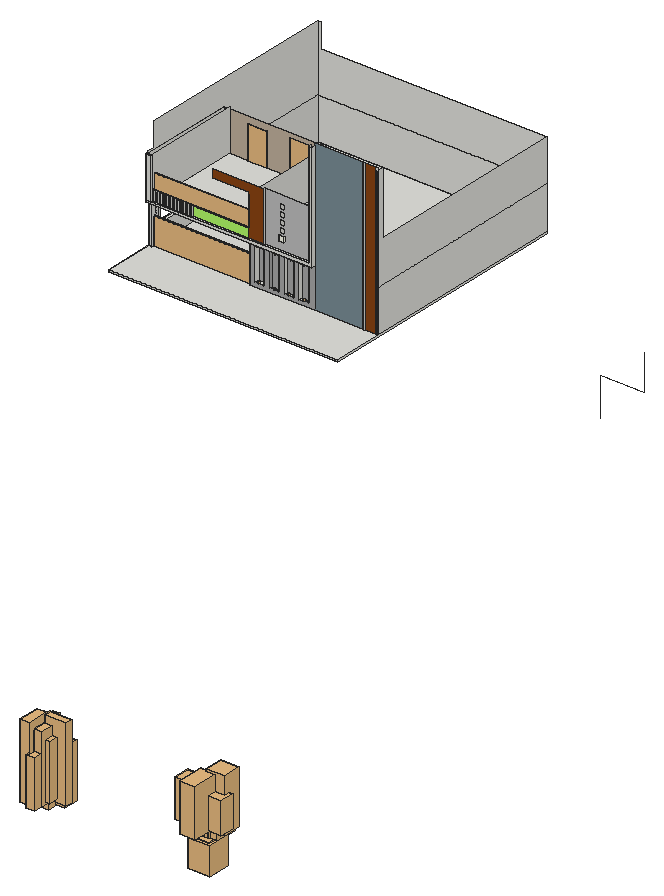
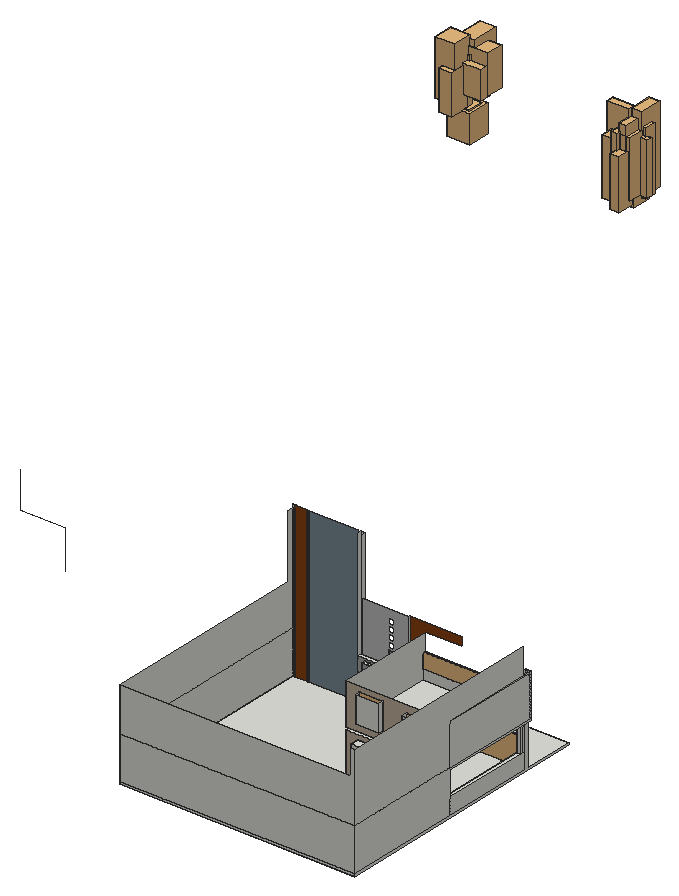
# SketchUp Ruby script. Lengths in inches.
U = 1.inch
M = Sketchup.active_model
def pt(a) = Geom::Point3d.new(a.map { |v| v * U })
def face(e, loops, mat)
  f = e.add_face(loops[0].map { |a| pt(a) })
  loops[1..].each { |l| e.add_face(l.map { |a| pt(a) }).erase! }
  f.material = f.back_material = mat if mat
  f
end
# faces: each face lists its corners as indices into pts; further lists are holes
def faces(e, pts, list, mat = nil) = list.each { |f| face(e, (f[0].is_a?(Array) ? f : [f]).map { |l| l.map { |i| pts[i] } }, mat) }
# xy, xz, yz: faces in a plane at the given z, y or x. An outline is a flat list of corners, or four numbers for a rectangle; further outlines are holes
def ring(l) = l.size == 4 ? [[l[0], l[1]], [l[2], l[1]], [l[2], l[3]], [l[0], l[3]]] : l.each_slice(2).to_a
def flat(e, list, mat, &to3) = list.each { |f| face(e, (f[0].is_a?(Array) ? f : [f]).map { |l| ring(l).map { |u, v| to3.(u, v) } }, mat) }
def xy(e, z, list, mat = nil) = flat(e, list, mat) { |x, y| [x, y, z] }
def xz(e, y, list, mat = nil) = flat(e, list, mat) { |x, z| [x, y, z] }
def yz(e, x, list, mat = nil) = flat(e, list, mat) { |y, z| [x, y, z] }
def lines(e, pts, list) = list.each { |a, b| e.add_line(pt(pts[a]), pt(pts[b])) }
# prism: a flat outline (further loops are holes) pulled along v
def prism(e, loops, v, mat = nil)
  f = face(e, loops, mat); d = Geom::Vector3d.new(v.map { |x| x * U })
  f.pushpull(f.normal.samedirection?(d) ? d.length : -d.length)
end
def box(e, o, s, mat = nil) = prism(e, [[o, [o[0] + s[0], o[1], o[2]], [o[0] + s[0], o[1] + s[1], o[2]], [o[0], o[1] + s[1], o[2]]]], [0, 0, s[2]], mat)
def at(x, y, z, deg = 0) = Geom::Transformation.translation(pt([x, y, z])) * Geom::Transformation.rotation(ORIGIN, Z_AXIS, deg.degrees)
def axes(o, x, y, z) = Geom::Transformation.new([*x, 0, *y, 0, *z, 0, *pt(o).to_a, 1])
def part(name) = M.definitions.add(name)
# library, detail: a bought-in or finely detailed component or shape, given as its bounding box
def library(name, o, s) = part(name).tap { |d| box(d.entities, o, s) }
def detail(e, o, s) = box(e.add_group.entities, o, s)
def put(e, d, t, mat = nil) = e.add_instance(d, t).tap { |i| i.material = mat if mat }
def group(e, t, mat = nil) = e.add_group.tap { |g| g.transformation = t; g.material = mat if mat }.entities
root = M.entities
M.materials.add("BANANA_BIG_STVOL_1").color = [93, 83, 53]
M.materials.add("POT_TEXTURE_1").color = [172, 172, 172]
M.materials.add("POT_TEXTURE_2").color = [160, 154, 144]
M.materials.add("[0043_SaddleBrown]").color = [139, 69, 19]
M.materials.add("[0053_Ivory]").color = [255, 255, 240]
M.materials.add("[0131_Silver]").color = [192, 192, 192]
M.materials.add("[Color F02]").color = [181, 255, 107]
M.materials.add("[Color M03]").color = [170, 170, 170]
M.materials.add("[Square Glass Tile 01]1").color = [123, 142, 151]
M.materials.add("[Tile Large Brown]").color = [195, 178, 159]
M.materials.add("soil1").color = [68, 55, 47]
M.materials.add("white_concrete_pot1").color = [212, 211, 204]
c1 = library("Group\#5",[-568.09,-2386.9,-3.76],[573.62,569.18,700.28])
c2 = library("Group\#35",[-480.58,1843.32,11.96],[467.85,466.24,378.92])
c3 = library("Single Door-001",[0,-7.11,0],[43.31,7.11,78.74])
c4 = library("DR 0003",[0,-1.57,0],[119.37,3.14,98.43])
c5 = library("Group\#60",[-273.21,1593.22,47.51],[374.54,419.07,1416.6])
c6 = library("Group\#59",[-208.23,2037.18,75.37],[621.09,225.61,1251.82])
c7 = library("Group\#65",[-231.77,1913.24,119.96],[448.93,143.84,1582.05])
c8 = library("Lamp Ceiling 114-44",[-1.26,-1.26,-3.9375],[2.52,2.52,3.9375])
c9 = library("Group\#61",[-527.15,2088.47,150.96],[267.01,328.12,1599.25])
c10 = library("Group\#68",[-792.12,2067.32,152.13],[549.56,259.52,1931.8])
c11 = library("Group\#62",[-675.58,1862.05,152.55],[378.81,196.01,1743.84])
c12 = library("Group\#56",[-904.81,1865.01,156.3],[624.43,217.34,1227.7])
c13 = library("Group\#63",[-257.06,2048.08,160.05],[394.6,177.93,1743.83])
c14 = library("Group\#64",[-344.84,1500.61,160.55],[176.35,551.19,1921.45])
c15 = library("Group\#66",[-616.67,2098.6,178.29],[331.19,111.16,1177.92])
c16 = library("Group\#58",[-571.16,1736.08,232.33],[294.08,306.57,1438.75])
c17 = library("Group\#67",[-236.03,2064.57,238.29],[378.97,266.89,1422.96])
c18 = library("Group\#69",[-281.17,2118.67,243.77],[133.23,408.71,1313.3])
c19 = library("Group\#57",[-312.51,1611.52,263.78],[120.52,408.52,1275.1])
c20 = library("Group\#12",[-392.38,2142.99,345.23],[79.77,60.6,39.05])
c21 = library("Group\#19",[-435.875,2067.96,347.82],[58.32,80.53,38.29])
c22 = library("Group\#20",[-362.86,1963.26,351.01],[55.56,80.44,37.9])
c23 = library("Group\#50",[-275.5,2156.34,352.11],[71.39,73.27,44.69])
c24 = library("Group\#38",[-363.89,1895.22,354.63],[76.92,66.54,39.48])
c25 = library("Group\#40",[-419.21,1941.11,355.02],[73.1,71.21,39.06])
c26 = library("Group\#16",[-389.63,2051.04,359.41],[56.81,81.38,37.86])
c27 = library("Group\#53",[-366.3125,2177.8,359.41],[79.9,61.23,37.86])
c28 = library("Group\#27",[-340.96,1970.4,361.28],[81.22,51.59,61.62])
c29 = library("Group\#39",[-390.04,2074.71,363.78],[77.3,84.83,61.55])
c30 = library("Group\#55",[-431.9,1883.46,368.72],[373.65,376.39,18.61])
c31 = library("Group\#13",[-433.57,2042.61,369.7],[71.79,72.8,37.85])
c32 = library("Group\#14",[-374.28,1979.7,369.99],[51.81,82.66,37.9])
c33 = library("Group\#22",[-330.83,2117.69,370.2],[61.83,80.2,35.55])
c34 = library("Group\#142",[-312.76,2118.02,370.79],[80.37,61.43,57.53])
c35 = library("Group\#47",[-315.77,2202.04,371],[80.74,54.44,37.85])
c36 = library("Group\#45",[-397.18,1916.74,372.44],[70.02,74.57,49.25])
c37 = library("Group\#15",[-432.01,1984.38,372.6875],[64.1,75.95,39.0625])
c38 = library("Group\#49",[-372.4375,2154.5,374],[76.125,67.08,39.0625])
c39 = library("Window",[191.41,-50.77,0.18],[4.75,0.44,6.52])
c40 = library("Group\#131",[-330.26,-2159.14,612.04],[116.66,119.22,673.97])
c41 = library("Group\#129",[-336.38,-2175.79,614.41],[133.99,147.1,560.64])
c42 = library("Group\#130",[-311.45,-2362.85,663.67],[597.01,322.07,1007.38])
c43 = library("Group\#128",[-480.3,-2300.47,677.45],[398.14,398.43,28.25])
c44 = part("Group186\#1")
p = [[0,0,0],[0,0,-1.62],[-0.6,0,-1.62],[3.88,-1.36,0],[-3.88,-1.36,0],[3.88,1.36,0],
  [3.88,0,0],[-3.88,1.36,0],[0.6,0,-1.62],[-3.88,0,0],[0,0,-2.62]]
lines(c44.entities,p,[[0,1],[1,2],[3,4],[5,6],[7,5],[1,8],[9,0],[0,6],[8,10],[4,9],[6,3],[2,10],
  [9,7]])
c45 = part("Rectangle Light")
put(c45.entities,c44,at(0,0,0))
c46 = library("Group\#138",[-308.37,-2556.11,869.35],[483.58,483.6,1385.8])
c47 = library("Group\#134",[-943.22,-2312.1875,967.59],[670.63,402.45,1245.73])
c48 = library("Group\#136",[-343.93,-2076.42,1024.91],[285.05,475.82,708.21])
c49 = library("Group\#137",[-550.09,-2664.39,1031.96],[371.42,533.86,798])
c50 = library("Group\#132",[-667.53,-2111.4375,1071.74],[420.02,555.28,968.03])
c51 = library("Aluprof_MB-86_Drzwi_panelowe_003_S-0452",[0,0,0],[44.84,5.36,87])
c52 = library("Group\#133",[-328.97,-2115.58,1156.29],[117.86,119.42,695.38])
c53 = library("Wagner Glass Railing",[9.08,102.375,1.53],[2.51,145.5,42.05])
xy(root,-6,[[0,1983.76,651.875,2725.58]])
xy(root,0,[[0,1983.76,651.875,1983.76,651.875,2124.78,645.875,2124.78,645.875,2125.58,613.45,2125.58,613.45,2124.78,608.45,2124.78,608.45,2125.58,287.74,2125.58,287.74,2396.39,131.5,2396.39,131.5,2418.76,84.19,2418.76,84.19,2396.39,10.5625,2396.39,10.5625,2125.58,0,2125.58],[608.45,2124.78,613.45,2125.58],[608.45,2124.78,613.45,2125.58],[645.875,2124.78,651.875,2125.58],[287.74,2125.58,651.875,2125.58,651.875,2725.58,0,2725.58,0,2396.39,84.19,2396.39,84.19,2418.76,131.5,2418.76,131.5,2396.39,287.74,2396.39],
  [0,2138.22,10.5625,2396.39]])
xy(root,11.59,[[302.72,2125.58,328.6,2138.2],[344.47,2125.58,370.35,2131.64],[386.22,2125.58,412.1,2132.33],[427.97,2125.58,453.85,2134.14]])
xy(root,44.51,[[181.49,2396.39,254.93,2420.08]])
xy(root,46.375,[[0,2138.22,10.5625,2144.66],[0,2144.66,10.5625,2152.16],[0,2152.16,10.5625,2396.39]])
xy(root,98.1875,[[84.19,2396.39,131.5,2418.76]])
xy(root,99.76,[[181.49,2396.39,254.93,2420.08]])
xy(root,105.15,[[302.72,2125.58,328.6,2138.2],[344.47,2125.58,370.35,2131.64],[386.22,2125.58,412.1,2132.33],[427.97,2125.58,453.85,2134.14]])
xy(root,113,[[0,2115.7,0,2125.58,10.5625,2125.58,10.5625,2152.16,0,2152.16,0,2396.39,287.74,2396.39,287.74,2125.58,472.61,2125.58,472.61,2115.7],[0,2138.22,10.5625,2144.66],[0,2144.66,10.5625,2152.16]])
xy(root,120,[[0,2115.7,12.86,2119.76],[12.86,2115.7,461.86,2115.7,461.86,2125.58,329.67,2125.58,329.67,2123.01,128.4,2123.01,128.4,2120.01,121.85,2120.01,121.85,2123.01,116.32,2123.01,116.32,2120.01,109.77,2120.01,109.77,2123.01,104.23,2123.01,104.23,2120.01,97.68,2120.01,97.68,2123.01,92.15,2123.01,92.15,2120.01,85.6,2120.01,85.6,2123.01,80.07,2123.01,80.07,2120.01,73.52,2120.01,73.52,2123.01,67.98,2123.01,67.98,2120.01,61.43,2120.01,61.43,2123.01,55.9,2123.01,55.9,2120.01,49.35,2120.01,49.35,2123.01,43.82,2123.01,43.82,2120.01,37.27,2120.01,37.27,2123.01,31.73,2123.01,31.73,2120.01,25.18,2120.01,25.18,2123.01,19.65,2123.01,19.65,2120.01,12.86,2120.01],[0,2119.76,12.86,2396.39],[12.86,2120.01,19.65,2123.01],[25.18,2120.01,31.73,2123.01],
  [37.27,2120.01,43.82,2123.01],[49.35,2120.01,55.9,2123.01],[61.43,2120.01,67.98,2123.01],[73.52,2120.01,80.07,2123.01],[85.6,2120.01,92.15,2123.01],
  [97.68,2120.01,104.23,2123.01],[109.77,2120.01,116.32,2123.01],[121.85,2120.01,128.4,2123.01],[12.86,2130.01,287.74,2130.01,287.74,2396.39,119.53,2396.39,119.53,2414.64,67.09,2414.64,67.09,2396.39,12.86,2396.39]])
xy(root,142.73,[[371.76,2122.39,386.07,2125.58]],"[0053_Ivory]")
xy(root,146.37,[[185.8,2396.39,250.98,2410.14]])
xy(root,146.875,[[12.86,2120.01,19.65,2123.01],[25.18,2120.01,31.73,2123.01],[37.27,2120.01,43.82,2123.01],[49.35,2120.01,55.9,2123.01],[61.43,2120.01,67.98,2123.01],
  [73.52,2120.01,80.07,2123.01],[85.6,2120.01,92.15,2123.01],[97.68,2120.01,104.23,2123.01],[109.77,2120.01,116.32,2123.01],[121.85,2120.01,128.4,2123.01],
  [12.86,2123.01,287.74,2130.01]])
xz(root,1983.76,[[0,-6,651.875,0]])
xz(root,2115.7,[[0,113,472.61,113,472.61,417.125,461.86,417.125,461.86,120,0,120],[0,120,12.86,236.3125]])
xz(root,2119.76,[[0,120,12.86,236.3125]])
xz(root,2120.01,[[12.86,120,19.65,146.875],[25.18,120,31.73,146.875],[37.27,120,43.82,146.875],[49.35,120,55.9,146.875],[61.43,120,67.98,146.875],
  [73.52,120,80.07,146.875],[85.6,120,92.15,146.875],[97.68,120,104.23,146.875],[109.77,120,116.32,146.875],[121.85,120,128.4,146.875]])
xz(root,2122.39,[[371.76,142.73,386.07,157.04]],"[0053_Ivory]")
xz(root,2123.01,[[12.86,120,19.65,146.875],[25.18,120,31.73,146.875],[37.27,120,43.82,146.875],[49.35,120,55.9,146.875],[61.43,120,67.98,146.875],
  [73.52,120,80.07,146.875],[85.6,120,92.15,146.875],[97.68,120,104.23,146.875],[109.77,120,116.32,146.875],[121.85,120,128.4,146.875]])
xz(root,2123.01,[[287.74,120,329.67,120,329.67,260.25,185.58,260.25,185.58,236.3125,287.74,236.3125]],"[0043_SaddleBrown]")
xz(root,2123.01,[[19.65,120,25.18,146.875],[31.73,120,37.27,146.875],[43.82,120,49.35,146.875],[55.9,120,61.43,146.875],[67.98,120,73.52,146.875],
  [80.07,120,85.6,146.875],[92.15,120,97.68,146.875],[104.23,120,109.77,146.875],[116.32,120,121.85,146.875],[128.4,120,287.74,146.875]],"[Color F02]")
xz(root,2124.78,[[608.45,0,613.45,425.125],[645.875,0,651.875,425.125]])
xz(root,2125.58,[[0,0,10.5625,113],[608.45,0,613.45,425.125],[645.875,0,651.875,425.125]])
xz(root,2125.58,[[613.45,0,645.875,425.125]],"[0043_SaddleBrown]")
xz(root,2125.58,[[[329.67,120,461.86,260.25],[371.76,222.86,386.07,237.17],[371.76,202.82,386.07,217.14],[371.76,182.79,386.07,197.11],[371.76,162.76,386.07,177.07],[371.76,142.73,386.07,157.04]],[371.76,142.73,386.07,157.04]],"[0131_Silver]")
xz(root,2125.58,[[[287.74,0,472.61,113],[302.72,11.59,328.6,105.15],[344.47,11.59,370.35,105.15],[386.22,11.59,412.1,105.15],[427.97,11.59,453.85,105.15]]],"[Color M03]")
xz(root,2125.58,[[472.61,0,608.45,425.125]],"[Square Glass Tile 01]1")
xz(root,2130.01,[[12.86,120,287.74,146.875]])
xz(root,2131.64,[[344.47,11.59,370.35,105.15]],"[Color M03]")
xz(root,2132.33,[[386.22,11.59,412.1,105.15]],"[Color M03]")
xz(root,2134.14,[[427.97,11.59,453.85,105.15]],"[Color M03]")
xz(root,2138.2,[[302.72,11.59,328.6,105.15]],"[Color M03]")
xz(root,2138.22,[[0,0,10.5625,46.375],[0,46.375,10.5625,113]])
xz(root,2144.66,[[0,46.375,10.5625,113]])
xz(root,2152.16,[[0,46.375,10.5625,113]])
xz(root,2396.39,[[0,0,10.5625,46.375],[0,120,12.86,233]])
xz(root,2396.39,[[[10.5625,0,84.19,0,84.19,98.1875,131.5,98.1875,131.5,0,287.74,0,287.74,113,0,113,0,46.375,10.5625,46.375],[181.49,44.51,254.93,99.76]],[[12.86,120,67.09,120,67.09,213,119.53,213,119.53,120,287.74,120,287.74,233,12.86,233],[185.8,146.37,250.98,219.25]]],"[Tile Large Brown]")
xz(root,2410.14,[[185.8,146.37,250.98,219.25]])
xz(root,2414.64,[[67.09,120,119.53,213]])
xz(root,2418.76,[[84.19,0,131.5,98.1875]])
xz(root,2420.08,[[181.49,44.51,254.93,99.76]])
xz(root,2725.58,[[0,-6,651.875,0],[0,0,651.875,120],[0,120,0,308.3125,10.1875,308.3125,10.1875,240,651.875,240,651.875,120]])
yz(root,0,[[1983.76,-6,1983.76,0,2125.58,0,2125.58,113,2138.22,113,2138.22,0,2725.58,0,2725.58,-6],[2396.39,0,2396.39,113,2115.7,113,2115.7,120,2725.58,120,2725.58,0],[2138.22,0,2396.39,46.375],[2138.22,46.375,2144.66,113],[2144.66,46.375,2152.16,113],
  [2115.7,120,2115.7,236.3125,2117.95,236.3125,2117.95,229.625,2119.76,229.625,2119.76,120],[2119.76,120,2119.76,229.625,2128.01,229.625,2128.01,233,2396.39,233,2396.39,120],[2396.39,120,2396.39,236.3125,2123.01,236.3125,2123.01,240,2143.83,240,2143.83,308.3125,2725.58,308.3125,2725.58,120]])
yz(root,10.5625,[[2125.58,0,2138.22,113],[2138.22,0,2396.39,46.375],[2138.22,46.375,2144.66,113],[2144.66,46.375,2152.16,113]])
yz(root,12.86,[[2115.7,120,2119.76,236.3125],[2119.76,120,2120.01,120,2120.01,146.875,2130.01,146.875,2130.01,120,2396.39,120,2396.39,236.3125,2119.76,236.3125],[2120.01,120,2123.01,146.875],[2123.01,120,2130.01,146.875]])
yz(root,19.65,[[2120.01,120,2123.01,146.875]])
yz(root,25.18,[[2120.01,120,2123.01,146.875]])
yz(root,31.73,[[2120.01,120,2123.01,146.875]])
yz(root,37.27,[[2120.01,120,2123.01,146.875]])
yz(root,43.82,[[2120.01,120,2123.01,146.875]])
yz(root,49.35,[[2120.01,120,2123.01,146.875]])
yz(root,55.9,[[2120.01,120,2123.01,146.875]])
yz(root,61.43,[[2120.01,120,2123.01,146.875]])
yz(root,67.09,[[2396.39,120,2414.64,213]])
yz(root,67.98,[[2120.01,120,2123.01,146.875]])
yz(root,73.52,[[2120.01,120,2123.01,146.875]])
yz(root,80.07,[[2120.01,120,2123.01,146.875]])
yz(root,84.19,[[2396.39,0,2418.76,98.1875]])
yz(root,85.6,[[2120.01,120,2123.01,146.875]])
yz(root,92.15,[[2120.01,120,2123.01,146.875]])
yz(root,97.68,[[2120.01,120,2123.01,146.875]])
yz(root,104.23,[[2120.01,120,2123.01,146.875]])
yz(root,109.77,[[2120.01,120,2123.01,146.875]])
yz(root,116.32,[[2120.01,120,2123.01,146.875]])
yz(root,119.53,[[2396.39,120,2414.64,213]])
yz(root,121.85,[[2120.01,120,2123.01,146.875]])
yz(root,128.4,[[2120.01,120,2123.01,146.875]])
yz(root,131.5,[[2396.39,0,2418.76,98.1875]])
yz(root,181.49,[[2396.39,44.51,2420.08,99.76]])
yz(root,185.8,[[2396.39,146.37,2410.14,219.25]])
yz(root,250.98,[[2396.39,146.37,2410.14,219.25]])
yz(root,254.93,[[2396.39,44.51,2420.08,99.76]])
yz(root,287.74,[[2125.58,0,2396.39,113],[2130.01,120,2130.01,146.875,2123.01,146.875,2123.01,229.625,2128.01,229.625,2128.01,233,2396.39,233,2396.39,120]])
yz(root,302.72,[[2125.58,11.59,2138.2,105.15]])
yz(root,328.6,[[2125.58,11.59,2138.2,105.15]],"[Color M03]")
yz(root,329.67,[[2123.01,120,2125.58,260.25]])
yz(root,344.47,[[2125.58,11.59,2131.64,105.15]],"[Color M03]")
yz(root,370.35,[[2125.58,11.59,2131.64,105.15]],"[Color M03]")
yz(root,371.76,[[2122.39,142.73,2125.58,157.04]],"[0053_Ivory]")
yz(root,386.07,[[2122.39,142.73,2125.58,157.04]],"[0053_Ivory]")
yz(root,386.22,[[2125.58,11.59,2132.33,105.15]])
yz(root,412.1,[[2125.58,11.59,2132.33,105.15]],"[Color M03]")
yz(root,427.97,[[2125.58,11.59,2134.14,105.15]])
yz(root,453.85,[[2125.58,11.59,2134.14,105.15]],"[Color M03]")
yz(root,461.86,[[2115.7,120,2125.58,416.5]])
yz(root,472.61,[[2115.7,113,2125.58,417.125]])
yz(root,608.45,[[2124.78,0,2125.58,425.125]])
yz(root,613.45,[[2124.78,0,2125.58,425.125]])
yz(root,645.875,[[2124.78,0,2125.58,120],[2124.78,120,2125.58,417.125]])
yz(root,651.875,[[1983.76,-6,2725.58,0],[2124.78,0,2125.58,120],[2125.58,0,2725.58,120],[2124.78,120,2125.58,417.125],[2125.58,120,2725.58,120,2725.58,240,2143.83,240,2143.83,417.125,2125.58,417.125]])
p = [[1298.09,2107.36,23.67],[1298.09,2107.36,132.6],[1422.97,2107.36,132.6],[1422.97,2107.36,233.67]]
lines(root,p,[[0,1],[1,2],[2,3]])
put(root,c1,axes([1623.21,47.95,-4.19],[0,0.11,0],[-0.11,0,0],[0,0,0.11]),"POT_TEXTURE_2")
put(root,c2,axes([1623.21,47.95,-4.19],[0,0.11,0],[-0.11,0,0],[0,0,0.11]),"POT_TEXTURE_1")
put(root,c3,axes([84.19,2402.6875,0],[1.11,0,0],[0,0.77119,0],[0,0,1.2441]))
put(root,c4,axes([10.5625,2131.9,0],[2.32197,0,0],[0,1,0],[0,0,0.78]))
put(root,c5,axes([1623.21,47.95,-4.19],[0,0.11,0],[-0.11,0,0],[0,0,0.11]))
put(root,c6,axes([1623.21,47.95,-4.19],[0,0.11,0],[-0.11,0,0],[0,0,0.11]))
put(root,c7,axes([1623.21,47.95,-4.19],[0,0.11,0],[-0.11,0,0],[0,0,0.11]))
put(root,c8,axes([397.9,2126.84,11.59],[-1,0,0],[0,1,0],[0,0,-1]))
put(root,c8,axes([439.65,2126.84,11.59],[-1,0,0],[0,1,0],[0,0,-1]))
put(root,c8,axes([311.65,2126.84,11.59],[-1,0,0],[0,1,0],[0,0,-1]))
put(root,c8,axes([356.15,2126.84,11.59],[-1,0,0],[0,1,0],[0,0,-1]))
put(root,c9,axes([1623.21,47.95,-4.19],[0,0.11,0],[-0.11,0,0],[0,0,0.11]))
put(root,c10,axes([1623.21,47.95,-4.19],[0,0.11,0],[-0.11,0,0],[0,0,0.11]))
put(root,c11,axes([1623.21,47.95,-4.19],[0,0.11,0],[-0.11,0,0],[0,0,0.11]))
put(root,c12,axes([1623.21,47.95,-4.19],[0,0.11,0],[-0.11,0,0],[0,0,0.11]))
put(root,c13,axes([1623.21,47.95,-4.19],[0,0.11,0],[-0.11,0,0],[0,0,0.11]))
put(root,c14,axes([1623.21,47.95,-4.19],[0,0.11,0],[-0.11,0,0],[0,0,0.11]))
put(root,c15,axes([1623.21,47.95,-4.19],[0,0.11,0],[-0.11,0,0],[0,0,0.11]))
put(root,c16,axes([1623.21,47.95,-4.19],[0,0.11,0],[-0.11,0,0],[0,0,0.11]))
put(root,c17,axes([1623.21,47.95,-4.19],[0,0.11,0],[-0.11,0,0],[0,0,0.11]))
put(root,c18,axes([1623.21,47.95,-4.19],[0,0.11,0],[-0.11,0,0],[0,0,0.11]))
put(root,c19,axes([1623.21,47.95,-4.19],[0,0.11,0],[-0.11,0,0],[0,0,0.11]))
g1 = group(root,at(1623.21,47.95,-4.19),"white_concrete_pot1")
detail(g1,[-236.27,-35.13,37.31],[7.6,8.37,4.34])
g2 = group(root,at(1623.21,47.95,-4.19),"white_concrete_pot1")
detail(g2,[-248.44,-29.8,37.97],[9.02,5.73,4.21])
put(root,c20,axes([1623.21,47.95,-4.19],[0,0.11,0],[-0.11,0,0],[0,0,0.11]),"white_concrete_pot1")
put(root,c21,axes([1623.21,47.95,-4.19],[0,0.11,0],[-0.11,0,0],[0,0,0.11]),"white_concrete_pot1")
g3 = group(root,at(1623.21,47.95,-4.19),"white_concrete_pot1")
detail(g3,[-229.91,-47.9,38.58],[6.88,8.66,4.16])
put(root,c22,axes([1623.21,47.95,-4.19],[0,0.11,0],[-0.11,0,0],[0,0,0.11]),"white_concrete_pot1")
put(root,c23,axes([1623.21,47.95,-4.19],[0,0.11,0],[-0.11,0,0],[0,0,0.11]),"white_concrete_pot1")
put(root,c24,axes([1623.21,47.95,-4.19],[0,0.11,0],[-0.11,0,0],[0,0,0.11]),"white_concrete_pot1")
put(root,c25,axes([1623.21,47.95,-4.19],[0,0.11,0],[-0.11,0,0],[0,0,0.11]),"white_concrete_pot1")
put(root,c26,axes([1623.21,47.95,-4.19],[0,0.11,0],[-0.11,0,0],[0,0,0.11]),"white_concrete_pot1")
put(root,c27,axes([1623.21,47.95,-4.19],[0,0.11,0],[-0.11,0,0],[0,0,0.11]),"white_concrete_pot1")
g4 = group(root,at(1623.21,47.95,-4.19),"white_concrete_pot1")
detail(g4,[-231.14,-43.4,39.59],[7.13,8.76,4.09])
put(root,c28,axes([1623.21,47.95,-4.19],[0,0.11,0],[-0.11,0,0],[0,0,0.11]),"white_concrete_pot1")
put(root,c29,axes([1623.21,47.95,-4.19],[0,0.11,0],[-0.11,0,0],[0,0,0.11]),"white_concrete_pot1")
put(root,c30,axes([1623.21,47.95,-4.19],[0,0.11,0],[-0.11,0,0],[0,0,0.11]),"white_concrete_pot1")
put(root,c31,axes([1623.21,47.95,-4.19],[0,0.11,0],[-0.11,0,0],[0,0,0.11]),"white_concrete_pot1")
g5 = group(root,at(1623.21,47.95,-4.19),"white_concrete_pot1")
detail(g5,[-241.13,-45.94,40.68],[8.75,7.2,4.21])
put(root,c32,axes([1623.21,47.95,-4.19],[0,0.11,0],[-0.11,0,0],[0,0,0.11]),"white_concrete_pot1")
put(root,c33,axes([1623.21,47.95,-4.19],[0,0.11,0],[-0.11,0,0],[0,0,0.11]),"white_concrete_pot1")
put(root,c34,axes([1623.21,47.95,-4.19],[0,0.11,0],[-0.11,0,0],[0,0,0.11]),"white_concrete_pot1")
put(root,c35,axes([1623.21,47.95,-4.19],[0,0.11,0],[-0.11,0,0],[0,0,0.11]),"white_concrete_pot1")
put(root,c36,axes([1623.21,47.95,-4.19],[0,0.11,0],[-0.11,0,0],[0,0,0.11]),"white_concrete_pot1")
put(root,c37,axes([1623.21,47.95,-4.19],[0,0.11,0],[-0.11,0,0],[0,0,0.11]),"white_concrete_pot1")
put(root,c38,axes([1623.21,47.95,-4.19],[0,0.11,0],[-0.11,0,0],[0,0,0.11]),"white_concrete_pot1")
put(root,c39,axes([-2779.68,2556.27,42.95],[15.46994,0,0],[0,3.14877,0],[0,0,8.47727]))
put(root,c40,axes([1623.21,47.95,-4.19],[0,0.11,0],[-0.11,0,0],[0,0,0.11]),"BANANA_BIG_STVOL_1")
put(root,c41,axes([1623.21,47.95,-4.19],[0,0.11,0],[-0.11,0,0],[0,0,0.11]),"BANANA_BIG_STVOL_1")
put(root,c42,axes([1623.21,47.95,-4.19],[0,0.11,0],[-0.11,0,0],[0,0,0.11]))
put(root,c43,axes([1623.21,47.95,-4.19],[0,0.11,0],[-0.11,0,0],[0,0,0.11]),"soil1")
put(root,c45,axes([202.9,2420.07,77.25],[1,0,0],[0,0,-1],[0,1,0]))
put(root,c46,axes([1623.21,47.95,-4.19],[0,0.11,0],[-0.11,0,0],[0,0,0.11]))
put(root,c8,at(358.66,2126.84,105.15))
put(root,c8,at(441.35,2126.84,105.15))
put(root,c8,at(317.71,2133.21,105.15))
put(root,c8,at(401.75,2129.76,105.15))
put(root,c47,axes([1623.21,47.95,-4.19],[0,0.11,0],[-0.11,0,0],[0,0,0.11]))
put(root,c48,axes([1623.21,47.95,-4.19],[0,0.11,0],[-0.11,0,0],[0,0,0.11]))
put(root,c49,axes([1623.21,47.95,-4.19],[0,0.11,0],[-0.11,0,0],[0,0,0.11]))
put(root,c50,axes([1623.21,47.95,-4.19],[0,0.11,0],[-0.11,0,0],[0,0,0.11]))
put(root,c51,axes([67.09,2394.71,120],[1.19,0,0],[0,1,0],[0,0,1.06896]))
put(root,c52,axes([1623.21,47.95,-4.19],[0,0.11,0],[-0.11,0,0],[0,0,0.11]))
put(root,c39,axes([-2442.71,2624.28,144.31],[13.73204,0,0],[0,4.5,0],[0,0,11.18156]))
put(root,c53,axes([-180.55,2138.11,145.34],[0,-1,0],[1.88921,0,0],[0,0,1]))
